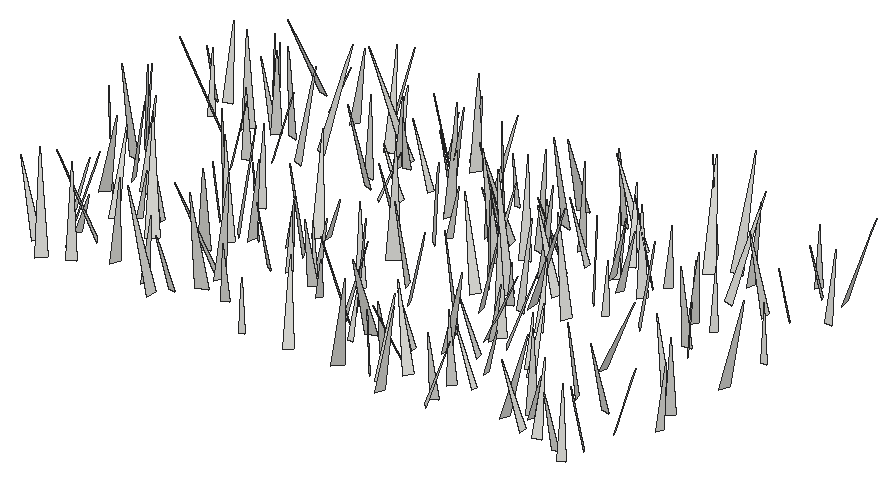
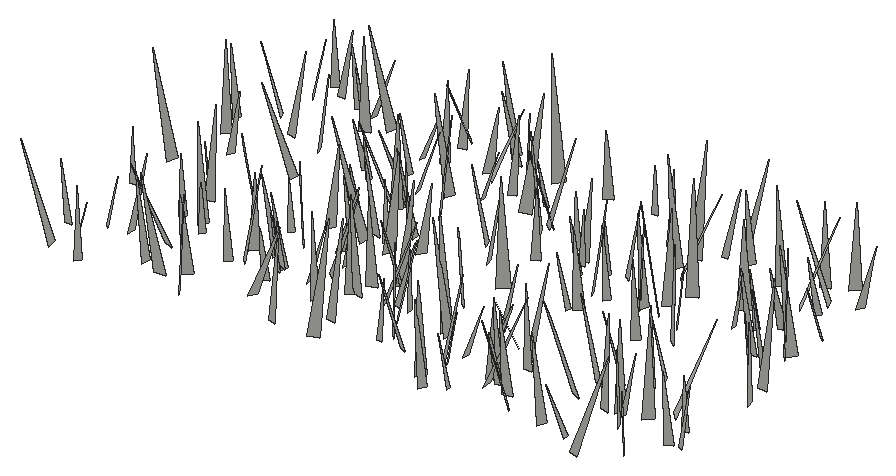
# SketchUp Ruby script. Lengths in inches.
U = 1.inch
M = Sketchup.active_model
def pt(a) = Geom::Point3d.new(a.map { |v| v * U })
def face(e, loops, mat)
  f = e.add_face(loops[0].map { |a| pt(a) })
  loops[1..].each { |l| e.add_face(l.map { |a| pt(a) }).erase! }
  f.material = f.back_material = mat if mat
  f
end
# faces: each face lists its corners as indices into pts; further lists are holes
def faces(e, pts, list, mat = nil) = list.each { |f| face(e, (f[0].is_a?(Array) ? f : [f]).map { |l| l.map { |i| pts[i] } }, mat) }
# xy, xz, yz: faces in a plane at the given z, y or x. An outline is a flat list of corners, or four numbers for a rectangle; further outlines are holes
def ring(l) = l.size == 4 ? [[l[0], l[1]], [l[2], l[1]], [l[2], l[3]], [l[0], l[3]]] : l.each_slice(2).to_a
def flat(e, list, mat, &to3) = list.each { |f| face(e, (f[0].is_a?(Array) ? f : [f]).map { |l| ring(l).map { |u, v| to3.(u, v) } }, mat) }
def xy(e, z, list, mat = nil) = flat(e, list, mat) { |x, y| [x, y, z] }
def xz(e, y, list, mat = nil) = flat(e, list, mat) { |x, z| [x, y, z] }
def yz(e, x, list, mat = nil) = flat(e, list, mat) { |y, z| [x, y, z] }
def lines(e, pts, list) = list.each { |a, b| e.add_line(pt(pts[a]), pt(pts[b])) }
# prism: a flat outline (further loops are holes) pulled along v
def prism(e, loops, v, mat = nil)
  f = face(e, loops, mat); d = Geom::Vector3d.new(v.map { |x| x * U })
  f.pushpull(f.normal.samedirection?(d) ? d.length : -d.length)
end
def box(e, o, s, mat = nil) = prism(e, [[o, [o[0] + s[0], o[1], o[2]], [o[0] + s[0], o[1] + s[1], o[2]], [o[0], o[1] + s[1], o[2]]]], [0, 0, s[2]], mat)
def at(x, y, z, deg = 0) = Geom::Transformation.translation(pt([x, y, z])) * Geom::Transformation.rotation(ORIGIN, Z_AXIS, deg.degrees)
def axes(o, x, y, z) = Geom::Transformation.new([*x, 0, *y, 0, *z, 0, *pt(o).to_a, 1])
def part(name) = M.definitions.add(name)
# library, detail: a bought-in or finely detailed component or shape, given as its bounding box
def library(name, o, s) = part(name).tap { |d| box(d.entities, o, s) }
def detail(e, o, s) = box(e.add_group.entities, o, s)
def put(e, d, t, mat = nil) = e.add_instance(d, t).tap { |i| i.material = mat if mat }
def group(e, t, mat = nil) = e.add_group.tap { |g| g.transformation = t; g.material = mat if mat }.entities
root = M.entities
c1 = part("fur_instance\#9")
p = [[0.8125,0,1.79],[0.67,-0.02,1.48],[0,-0.11,0],[0,0.11,0]]
faces(c1.entities,p,[[0,1,2,3]])
put(root,c1,axes([515.94,55.68,-21.66],[6.14943,-1.42717,1.61929],[-1.52874,-6.3314,0.22535],[-1.52376,0.59247,6.30885]))
put(root,c1,axes([507.93,57.48,-21.66],[6.18232,-5.30847,0.7026],[-5.32058,-6.21081,-0.10875],[-0.60412,0.37485,8.14795]))
put(root,c1,axes([544.28,55.85,-21.66],[-3.13208,3.88614,1.48189],[4.03166,3.29255,-0.11327],[1.02167,-1.07935,4.98991]))
put(root,c1,axes([542.07,57.4375,-21.66],[0.17037,-4.40384,1.04145],[-4.5148,-0.2364,-0.26107],[-0.30825,1.02847,4.3994]))
put(root,c1,axes([493.76,56.37,-21.66],[-0.42673,3.51272,1.26133],[3.73148,0.37463,0.21911],[-0.0791,-1.27778,3.53176]))
put(root,c1,axes([462.76,55.75,-21.66],[-5.4488,4.52209,1.619],[4.59694,5.6194,-0.22458],[1.39234,-0.85616,7.07731]))
put(root,c1,axes([479.05,57.01,-21.66],[-7.32255,-0.11088,1.35528],[-0.08815,7.44603,0.13288],[1.35695,-0.11461,7.32218]))
put(root,c1,axes([522.46,58.125,-21.66],[1.7038,-4.78318,1.39426],[-4.94528,-1.80274,-0.14134],[-0.60574,1.26373,5.0756]))
put(root,c1,axes([522.62,56.23,-21.66],[3.07177,3.42083,0.35758],[3.42072,-3.08846,0.16062],[-0.35863,-0.15826,4.59478]))
put(root,c1,axes([480.32,59.38,-21.66],[-0.08561,-4.51883,0.61864],[-4.55746,0.06047,-0.18896],[-0.17898,0.62161,4.51569]))
put(root,c1,axes([466.05,57.49,-21.66],[-2.20554,5.93145,2.00046],[6.2413,2.24627,0.22087],[0.47966,-1.95462,6.32437]))
put(root,c1,axes([500.67,56.875,-21.66],[-3.10471,5.12305,0.88051],[5.18598,3.12286,0.11631],[0.35573,-0.81381,5.98927]))
put(root,c1,axes([512.32,58.2,-21.66],[2.78644,2.89477,1.9564],[3.12581,-3.18339,0.25829],[-1.56092,-1.20736,4.00964]))
put(root,c1,axes([514.49,57.23,-21.66],[0.1573,5.82785,1.1486],[5.93788,-0.12389,-0.18455],[0.15705,-1.15268,5.82705]))
put(root,c1,axes([476.6,58.78,-21.66],[4.38951,-2.01268,1.547],[-2.15257,-4.58905,0.13732],[-1.34555,0.7756,4.82698]))
put(root,c1,axes([535.8,58.77,-21.66],[-4.77809,0.40303,0.49366],[0.4272,4.79644,0.21897],[0.47289,-0.2608,4.79006]))
put(root,c1,axes([544.7,59.71,-21.66],[-3.48684,-2.54111,1.02639],[-2.66037,3.53733,-0.28017],[0.65812,0.83597,4.30544]))
put(root,c1,axes([459.46,58.95,-21.66],[-4.99004,2.24313,0.58277],[2.2784,5.00139,0.2583],[0.42444,-0.4756,5.46492]))
put(root,c1,axes([538.38,58.38,-21.66],[-2.22109,4.73282,1.14399],[4.81333,2.32397,-0.26934],[0.73496,-0.91711,5.22114]))
put(root,c1,axes([531.96,60.09,-21.66],[6.74375,-1.56753,0.95704],[-1.61805,-6.79399,0.27364],[-0.86892,0.48558,6.91813]))
put(root,c1,axes([470.56,60.54,-21.66],[5.91489,-2.56905,1.81184],[-2.61095,-6.16477,-0.21752],[-1.75092,0.51416,6.44505]))
put(root,c1,axes([487.22,61.26,-21.66],[2.10827,-4.41232,0.88185],[-4.4927,-2.11805,0.1432],[-0.24874,0.85808,4.88803]))
put(root,c1,axes([482.97,61.99,-21.66],[2.46891,-7.20313,1.70316],[-7.36136,-2.57683,-0.22704],[-0.77207,1.53499,7.61111]))
put(root,c1,axes([514.81,62.16,-21.66],[-3.4454,-3.89131,0.03074],[-3.88746,3.44363,0.20759],[0.17579,-0.11462,5.19326]))
put(root,c1,axes([534.76,61.78,-21.66],[3.71508,-1.29272,0.27873],[-1.28155,-3.72443,-0.19222],[-0.32626,-0.0905,3.92887]))
put(root,c1,axes([462.98,60.62,-21.66],[6.72571,2.73267,0.89443],[2.78268,-6.75899,-0.27437],[-0.72399,-0.59256,7.25447]))
put(root,c1,axes([521.89,62.25,-21.66],[4.08918,-3.36848,1.98263],[-3.52303,-4.41912,-0.24183],[-1.69286,1.05996,5.29241]))
put(root,c1,axes([510.38,63.55,-21.66],[2.722,-4.21365,0.18087],[-4.20663,-2.72794,-0.24377],[-0.30292,0.01939,5.01046]))
put(root,c1,axes([465.27,63.52,-21.66],[-5.5722,-4.07145,0.43281],[-4.071,5.58734,0.1482],[0.43699,0.13539,6.89957]))
put(root,c1,axes([516.1,61,-21.66],[-4.785,3.6619,0.62252],[3.69492,4.79647,0.18627],[0.38032,-0.52686,6.02254]))
put(root,c1,axes([534.39,62.39,-21.66],[-1.98157,5.41612,3.08152],[6.10168,2.34277,-0.19399],[1.26474,-2.81671,5.76397]))
put(root,c1,axes([462.39,63.51,-21.66],[3.14021,-1.95272,0.11029],[-1.95573,-3.13292,0.21476],[0.01996,0.24059,3.6916]))
put(root,c1,axes([506.39,66.02,-21.66],[2.6634,-7.09113,0.13913],[-7.08626,-2.66678,-0.26525],[-0.29724,0.03689,7.57017]))
put(root,c1,axes([524.63,63.32,-21.66],[-3.98782,0.86871,0.11292],[0.87287,3.98492,0.16912],[0.07423,-0.18933,4.07783]))
put(root,c1,axes([505.36,63.11,-21.66],[0.0321,3.78164,0.61426],[3.82721,-0.05969,0.16749],[-0.17489,-0.6122,3.77806]))
put(root,c1,axes([483.15,65.27,-21.66],[6.93717,-2.75986,2.51351],[-2.97128,-7.29338,0.19237],[-2.25967,1.11744,7.46352]))
put(root,c1,axes([481.44,66.5,-21.66],[-5.39414,-3.77764,0.22745],[-3.78403,5.38986,-0.22257],[0.05845,0.31282,6.58162]))
put(root,c1,axes([501.96,66.91,-21.66],[-3.86878,-4.9807,0.99535],[-5.05831,3.89149,-0.18804],[0.45997,0.9025,6.30392]))
put(root,c1,axes([544.89,65.53,-21.66],[4.65489,2.00226,0.76997],[2.06003,-4.68544,-0.26978],[-0.59848,-0.55448,5.06006]))
put(root,c1,axes([512.64,66.44,-21.66],[-3.89073,-0.42692,0.42553],[-0.44504,3.90915,-0.14719],[0.40654,0.19356,3.91132]))
put(root,c1,axes([523.32,67.25,-21.66],[3.83276,-0.80553,0.30542],[-0.78769,-3.84079,-0.24507],[-0.34886,-0.17786,3.90882]))
put(root,c1,axes([540.79,68.76,-21.66],[-1.08369,-5.40972,1.03151],[-5.49173,1.14023,0.21038],[0.41232,0.96864,5.51318]))
put(root,c1,axes([501.6,66.56,-21.66],[3.62165,4.35293,0.90177],[4.41878,-3.65214,-0.11732],[-0.48531,-0.76904,5.66132]))
put(root,c1,axes([477.28,69.61,-21.66],[4.02071,-6.30995,0.86141],[-6.36147,-4.02715,0.19326],[-0.29869,0.83076,7.47959]))
put(root,c1,axes([516.22,68.47,-21.66],[6.40795,-1.734,1.03011],[-1.73088,-6.48917,-0.15614],[-1.03535,0.11648,6.63658]))
put(root,c1,axes([495.57,69.25,-21.66],[2.79472,-2.37927,0.19168],[-2.37504,-2.80125,-0.14262],[-0.23842,0.01542,3.66757]))
put(root,c1,axes([458.3,67.97,-21.66],[2.21445,2.95218,0.72503],[3.03203,-2.20951,-0.26401],[-0.21871,-0.73996,3.68096]))
put(root,c1,axes([501.79,68.63,-21.66],[5.69134,3.55142,2.30083],[3.82093,-5.97012,-0.23634],[-1.81848,-1.42926,6.70433]))
put(root,c1,axes([535.89,69.44,-21.66],[4.40996,1.53054,2.75088],[1.88618,-5.07543,-0.19988],[-2.52036,-1.1203,4.66373]))
put(root,c1,axes([548.86,69.37,-21.66],[4.44334,-1.86269,1.64457],[-2.02269,-4.66849,0.17731],[-1.44323,0.80817,4.81471]))
put(root,c1,axes([520.02,69.99,-21.66],[-4.58656,-0.99691,0.53395],[-0.9871,4.61746,0.14195],[0.55187,-0.02624,4.69151]))
put(root,c1,axes([493.13,71.04,-21.66],[2.16413,-4.87719,1.14426],[-4.95965,-2.26151,-0.2591],[-0.70577,0.93721,5.32947]))
put(root,c1,axes([470.29,68.15,-21.66],[-5.1988,6.07272,1.14347],[6.1224,5.26442,-0.12263],[0.83765,-0.78798,7.99315]))
put(root,c1,axes([486.35,70.99,-21.66],[-2.7828,-3.97435,1.2381],[-4.07565,2.90431,0.16237],[0.84701,0.91751,4.84903]))
put(root,c1,axes([465.95,71.1,-21.66],[3.13443,-2.25979,0.73802],[-2.32723,-3.16608,0.18952],[-0.4851,0.5876,3.85946]))
put(root,c1,axes([463.53,68.97,-21.66],[-2.14385,5.53708,0.23418],[5.53457,2.15208,-0.21752],[0.2875,-0.13964,5.93364]))
put(root,c1,axes([528.35,69.8,-21.66],[-1.52341,4.48001,0.30788],[4.47725,1.54034,-0.26007],[0.34571,-0.20714,4.72479]))
put(root,c1,axes([492.76,71.94,-21.66],[-0.42877,3.87256,1.55947],[4.17346,0.35848,0.25729],[-0.1042,-1.57711,3.88772]))
put(root,c1,axes([526.67,71.23,-21.66],[-1.83169,3.1238,0.57494],[3.14275,1.87858,-0.19441],[0.4602,-0.39568,3.61599]))
put(root,c1,axes([468.62,72.25,-21.66],[-3.8802,0.07929,1.10053],[0.11582,4.03064,0.11798],[1.09728,-0.14508,3.87922]))
put(root,c1,axes([488.75,71.93,-21.66],[-3.06481,2.41196,1.362],[2.48233,3.29293,-0.24563],[1.22908,-0.63618,3.89234]))
put(root,c1,axes([458.44,73.67,-21.66],[5.57249,-4.36069,0.56036],[-4.38496,-5.5781,0.19774],[-0.31889,0.50141,7.07313]))
put(root,c1,axes([547.42,73.18,-21.66],[-3.8078,3.44308,3.43375],[4.19662,4.52997,0.11149],[2.45637,-2.40193,5.13242]))
put(root,c1,axes([513.98,73.22,-21.66],[-6.04607,-3.24149,2.31572],[-3.3744,6.40425,0.15438],[2.11738,0.95032,6.85845]))
put(root,c1,axes([478.23,73.08,-21.66],[-4.52139,5.22079,2.42729],[5.56937,4.74843,0.161],[1.45961,-1.94607,6.90462]))
put(root,c1,axes([459.07,74.31,-21.66],[-4.9247,-5.05159,2.9073],[-5.39927,5.38751,0.21521],[2.19519,1.91829,7.05159]))
put(root,c1,axes([518.82,74.01,-21.66],[4.01363,-0.60213,1.19124],[-0.70216,-4.16285,0.26162],[-1.13516,0.446,4.0501]))
put(root,c1,axes([491.41,74.21,-21.66],[3.83893,-0.81047,1.08867],[-0.8917,-3.9684,0.19003],[-1.0232,0.41758,3.91895]))
put(root,c1,axes([518.03,73.83,-21.66],[5.44846,0.74036,0.07595],[0.73692,-5.44519,0.21553],[-0.10422,0.20337,5.4943]))
put(root,c1,axes([521.3,73.87,-21.66],[4.74716,3.3592,0.52437],[3.38285,-4.75689,-0.1518],[-0.33985,-0.42721,5.81349]))
put(root,c1,axes([480.22,75.41,-21.66],[5.9168,-1.45412,1.7202],[-1.44139,-6.15974,-0.24915],[-1.73089,0.15879,6.08776]))
put(root,c1,axes([498.02,74.4,-21.66],[2.13883,-4.28297,3.06723],[-5.00629,-2.68295,-0.2554],[-1.63976,2.60467,4.7805]))
put(root,c1,axes([505.16,74.95,-21.66],[5.01565,1.80166,1.23073],[1.89818,-5.12441,-0.23415],[-1.07592,-0.64182,5.32428]))
put(root,c1,axes([480.64,75.9,-21.66],[-3.25997,-4.21096,1.97124],[-4.4396,3.53441,0.20814],[1.38129,1.42168,5.3213]))
put(root,c1,axes([484.92,76.76,-21.66],[3.8804,-2.67072,0.47699],[-2.66948,-3.90717,-0.15997],[-0.48385,0.13783,4.70793]))
put(root,c1,axes([487.4,76.46,-21.66],[-5.57513,-2.9786,1.92177],[-3.03694,5.86084,0.2736],[1.82819,0.65252,6.315]))
put(root,c1,axes([519.27,75.08,-21.66],[-5.69,4.35692,2.08043],[4.49689,5.95288,-0.16772],[1.75752,-1.1258,7.16454]))
put(root,c1,axes([477.97,75.39,-21.66],[5.88152,4.86813,2.28116],[5.13014,-6.09312,-0.22398],[-1.60749,-1.63397,7.63157]))
put(root,c1,axes([473.96,76.7,-21.66],[-3.08736,-2.6391,1.38175],[-2.74426,3.29386,0.15946],[1.15895,0.7691,4.05847]))
put(root,c1,axes([534.06,76.74,-21.66],[6.32443,-0.86949,0.03215],[-0.87008,-6.31952,0.24926],[0.00213,0.25131,6.37905]))
put(root,c1,axes([462.55,76.25,-21.66],[-0.45657,6.34549,1.8425],[6.59681,0.54314,-0.23589],[0.37708,-1.81886,6.35752]))
put(root,c1,axes([543.77,76.92,-21.66],[-4.87029,1.64927,0.93909],[1.65484,4.95663,-0.12272],[0.92923,-0.18296,5.1405]))
put(root,c1,axes([502.15,78.37,-21.66],[-5.31437,-1.63311,1.48269],[-1.72892,5.48589,-0.1545],[1.36976,0.58821,5.55749]))
put(root,c1,axes([459.34,78.15,-21.66],[5.12051,1.66894,1.66295],[1.70709,-5.37015,0.13306],[-1.62376,-0.38277,5.38398]))
put(root,c1,axes([513.03,79.12,-21.66],[5.83146,1.27805,1.15338],[1.33487,-5.92923,-0.17895],[-1.08712,-0.42484,5.96719]))
put(root,c1,axes([472.03,80.09,-21.66],[3.78368,4.97369,3.03573],[5.56614,-4.15585,-0.12867],[-1.72376,-2.50217,6.24798]))
put(root,c1,axes([522,79.2,-21.66],[-1.31854,4.49628,0.43937],[4.51767,1.31381,0.11263],[0.01505,-0.45333,4.68427]))
put(root,c1,axes([456.17,82.26,-21.66],[-0.95753,-7.17721,1.84222],[-7.39469,1.0444,0.22542],[0.47406,1.79439,7.23729]))
put(root,c1,axes([487.26,81.5,-21.66],[3.61055,-0.61097,0.20103],[-0.59508,-3.6081,-0.27795],[-0.24409,-0.24103,3.65131]))
put(root,c1,axes([515.02,82.45,-21.66],[2.03296,-3.43324,0.36978],[-3.45285,-2.01606,0.26469],[0.04074,0.45292,3.9812]))
put(root,c1,axes([548.43,82.57,-21.66],[6.87118,-2.4682,1.14103],[-2.53265,-6.93781,0.24398],[-0.98977,0.61792,7.29696]))
put(root,c1,axes([486.15,80.77,-21.66],[-3.98192,5.65644,1.02142],[5.69703,4.04883,-0.21229],[0.76316,-0.7113,6.91418]))
put(root,c1,axes([476.07,82.22,-21.66],[-2.39493,4.93051,2.15105],[5.27679,2.61079,-0.10925],[1.04521,-1.88321,5.4803]))
put(root,c1,axes([496.72,82.32,-21.66],[4.92232,-5.34816,3.43981],[-5.97476,-5.37881,0.1869],[-2.17654,2.67018,7.26616]))
put(root,c1,axes([517.0625,81.81,-21.66],[1.06492,5.99669,1.55027],[6.17359,-1.15473,0.22589],[-0.50038,-1.48458,6.08632]))
put(root,c1,axes([509.93,81.82,-21.66],[-5.57386,3.34507,0.61319],[3.34749,5.6042,-0.14346],[0.5998,-0.19191,6.49898]))
put(root,c1,axes([517.41,83.75,-21.66],[8.28106,0.30024,0.90595],[0.31898,-8.32832,-0.15571],[-0.89952,-0.18935,8.28504]))
put(root,c1,axes([510.06,84.21,-21.66],[4.77754,4.17311,2.72058],[4.61145,-5.13068,-0.22808],[-1.8844,-1.97551,6.33938]))
put(root,c1,axes([522.66,83.89,-21.66],[-6.31107,2.62453,1.38258],[2.63294,6.45317,-0.23139],[1.36651,-0.31261,6.83112]))
put(root,c1,axes([513.21,84.08,-21.66],[-7.4138,3.10521,1.79195],[3.13289,7.61249,-0.22981],[1.74312,-0.47482,8.03455]))
put(root,c1,axes([456.03,84.6875,-21.66],[3.99026,4.07334,2.14881],[4.32029,-4.29562,0.12027],[-1.59518,-1.44473,5.70086]))
put(root,c1,axes([455.0625,86.07,-21.66],[-4.85936,-1.80324,2.4582],[-1.94231,5.39639,0.11902],[2.34986,0.73149,5.18178]))
put(root,c1,axes([539.9375,86.04,-21.66],[-2.43911,-2.15453,1.73505],[-2.51562,2.68975,-0.19638],[1.15067,1.31336,3.24849]))
put(root,c1,axes([538.45,87.67,-21.66],[0.4786,-6.17329,1.68247],[-6.39725,-0.42884,0.2463],[0.12453,1.69584,6.18692]))
put(root,c1,axes([525.85,87.54,-21.66],[-2.23187,2.81976,1.51549],[3.01775,2.4697,-0.15093],[1.06816,-1.08561,3.59298]))
put(root,c1,axes([466.8,87.88,-21.66],[4.26525,2.34746,1.0733],[2.44325,-4.34035,-0.2164],[-0.83252,-0.71113,4.86375]))
put(root,c1,axes([518.05,87.66,-21.66],[-5.4054,2.23783,0.44972],[2.26041,5.40869,0.2551],[0.31726,-0.40826,5.84475]))
put(root,c1,axes([530.82,87.88,-21.66],[-3.67972,-3.6806,3.42599],[-4.33109,4.47676,0.15761],[2.55458,2.28831,5.20214]))
put(root,c1,axes([498.01,88.61,-21.66],[3.30572,4.13092,2.03155],[4.38871,-3.58299,0.14433],[-1.38957,-1.489,5.28881]))
put(root,c1,axes([490.24,90.58,-21.66],[-1.40933,-4.17013,0.64925],[-4.20295,1.44894,0.18319],[0.38311,0.55526,4.39803]))
put(root,c1,axes([522.62,89.11,-21.66],[3.82157,4.19761,2.25189],[4.45533,-4.17126,0.21447],[-1.68552,-1.50865,5.67259]))
put(root,c1,axes([507.04,89.48,-21.66],[-7.37907,1.498,2.27835],[1.63074,7.6926,0.22378],[2.18531,-0.6822,7.52626]))
put(root,c1,axes([467.23,90.51,-21.66],[1.77747,-4.94769,1.74658],[-5.22789,-1.82695,0.145],[-0.44649,1.69476,5.25529]))
put(root,c1,axes([515.35,90.03,-21.66],[-3.60239,-0.15597,0.87969],[-0.19043,3.7046,-0.12301],[0.87288,0.16452,3.60367]))
put(root,c1,axes([548.5,90.3,-21.66],[-0.06677,3.94377,1.582],[4.24655,0.00562,0.16522],[-0.15123,-1.5834,3.94087]))
put(root,c1,axes([498.66,90.79,-21.66],[3.79566,-1.87078,0.73995],[-1.92959,-3.83243,0.2087],[-0.56925,0.51676,4.2265]))
put(root,c1,axes([513.58,90.52,-21.66],[6.28963,-0.96384,2.1084],[-1.07131,-6.61487,0.17192],[-2.05588,0.49827,6.36073]))
put(root,c1,axes([506.45,90.0625,-21.66],[2.03381,4.83721,0.83738],[4.90479,-2.04045,-0.1258],[-0.20703,-0.82108,5.24587]))
put(root,c1,axes([535.49,92.67,-21.66],[5.23742,-3.794,0.7561],[-3.79638,-5.28528,-0.22367],[-0.74406,0.26094,6.46336]))
put(root,c1,axes([515.09,93.07,-21.66],[-2.82637,-5.01502,0.69558],[-5.06125,2.81969,-0.23605],[0.13409,0.7222,5.75179]))
put(root,c1,axes([460.44,94.08,-21.66],[-5.16383,-5.19186,0.43743],[-5.2089,5.15828,-0.26709],[0.11856,0.49863,7.31773]))
put(root,c1,axes([469.76,92.46,-21.66],[4.69401,2.26049,0.88712],[2.32694,-4.7392,-0.23643],[-0.69438,-0.60059,5.20458]))
put(root,c1,axes([504,93.98,-21.66],[-1.28236,-4.10189,0.60594],[-4.14572,1.27987,-0.10961],[0.07509,0.61118,4.29626]))
put(root,c1,axes([523.41,93.34,-21.66],[4.86131,-2.02952,0.59697],[-2.06386,-4.87843,0.22145],[-0.46454,0.43544,5.26329]))
put(root,c1,axes([538.64,92.7,-21.66],[-2.37433,3.47563,1.70417],[3.72029,2.6012,-0.12184],[1.06942,-1.33243,4.20745]))
put(root,c1,axes([483.01,94.51,-21.66],[-2.27159,-6.08211,1.19958],[-6.16809,2.34544,0.21162],[0.62109,1.04786,6.48903]))
put(root,c1,axes([509.51,92.15,-21.66],[-2.53684,6.34204,1.9532],[6.60869,2.60398,0.12835],[0.60133,-1.86275,6.82939]))
put(root,c1,axes([486.03,92.73,-21.66],[2.19151,2.85606,0.09461],[2.85445,-2.18225,-0.24214],[0.13471,-0.22234,3.59182]))
put(root,c1,axes([510.63,95.16,-21.66],[2.81621,-4.35059,0.38195],[-4.36621,-2.81499,0.12899],[-0.09891,0.39082,5.18093]))
put(root,c1,axes([502.12,93.91,-21.66],[3.8396,0.83392,1.68617],[0.96833,-4.16197,-0.14664],[-1.61273,-0.51356,3.92638]))
put(root,c1,axes([505.58,94.53,-21.66],[-6.60705,-1.5953,0.55499],[-1.61141,6.62494,-0.14037],[0.50631,0.26714,6.79547]))
put(root,c1,axes([488.34,94.29,-21.66],[-3.79909,0.62191,0.11225],[0.62576,3.79759,0.13861],[0.08831,-0.15497,3.84716]))
put(root,c1,axes([526.51,93.88,-21.66],[-4.60516,3.74944,1.60687],[3.84875,4.79672,-0.16237],[1.35183,-0.88372,5.93628]))
put(root,c1,axes([472.625,93.79,-21.66],[2.70818,5.99392,1.73773],[6.22026,-2.74585,-0.22279],[-0.5051,-1.67756,6.57356]))
put(root,c1,axes([534.09,94.58,-21.66],[2.31719,-2.3997,1.71249],[-2.74416,-2.55172,0.13746],[-1.07739,1.33819,3.33302]))
put(root,c1,axes([520.69,95.32,-21.66],[4.88822,-0.89007,0.63341],[-0.87396,-4.92864,-0.18113],[-0.65546,-0.06625,4.96529]))
put(root,c1,axes([495.4,95.01,-21.66],[7.52534,-2.11015,2.94691],[-2.32099,-8.02168,0.183],[-2.78389,0.98374,7.81345]))
put(root,c1,axes([509.59,94.875,-21.66],[-1.17344,-6.36654,3.3674],[-7.15717,1.41187,0.17527],[0.80444,3.27459,6.4714]))
put(root,c1,axes([516.35,95.89,-21.66],[-4.66446,-0.17714,0.77084],[-0.14932,4.72517,0.1823],[0.77671,-0.15541,4.66426]))
put(root,c1,axes([494.57,95.84,-21.66],[7.78387,0.2727,2.09642],[0.3333,-8.05673,-0.18953],[-2.08764,-0.26953,7.78634]))
put(root,c1,axes([525.74,96.8,-21.66],[4.20893,3.73459,3.7879],[4.59902,-4.98198,-0.19834],[-2.67289,-2.69131,5.62342]))
put(root,c1,axes([501.75,96.77,-21.66],[-4.7875,-3.33897,1.34753],[-3.4677,4.87923,-0.23006],[0.96934,0.96392,5.83232]))
put(root,c1,axes([481.63,96.44,-21.66],[0.33576,5.45677,2.6197],[6.05197,-0.25349,-0.24764],[0.11336,-2.62894,5.46148]))
put(root,c1,axes([520.93,96.17,-21.66],[1.65832,3.59632,1.35209],[3.82471,-1.68517,-0.20869],[-0.36513,-1.31848,3.95475]))
put(root,c1,axes([462.46,96.79,-21.66],[-4.98307,4.13485,3.06586],[4.6284,5.46651,0.15019],[2.25263,-2.08511,6.47344]))
put(root,c1,axes([521.05,95.57,-21.66],[-1.86481,4.13252,0.34952],[4.14724,1.85655,0.17621],[-0.01744,-0.39104,4.53037]))
put(root,c1,axes([456.92,96.39,-21.66],[-1.17354,4.22506,1.16991],[4.38332,1.15287,0.2334],[0.0799,-1.19029,4.3788]))
put(root,c1,axes([466.07,97.78,-21.66],[4.61817,-3.87726,2.02523],[-4.05143,-4.90172,-0.14567],[-1.64942,1.18414,6.02822]))
put(root,c1,axes([527.37,97.9,-21.66],[-2.45808,3.26284,2.53045],[3.74921,2.99751,-0.22312],[1.72995,-1.86016,4.07903]))
put(root,c1,axes([468.05,98.375,-21.66],[-1.72933,-6.01967,2.37326],[-6.41752,1.90965,0.16749],[0.82719,2.23073,6.26091]))
put(root,c1,axes([465.38,98.1,-21.66],[-4.97388,0.03891,0.99351],[0.0174,5.07103,-0.11152],[0.99411,0.10595,4.97278]))
put(root,c1,axes([513.2,98.7,-21.66],[5.69837,-0.41307,2.53776],[-0.52377,-6.22748,0.16244],[-2.51724,0.36068,5.71101]))
put(root,c1,axes([489.6875,98.41,-21.66],[-4.67921,0.76999,0.1435],[0.76372,4.67821,-0.1991],[0.17382,0.17327,4.73796]))
put(root,c1,axes([454.9,99.89,-21.66],[-2.14945,-3.42966,1.0737],[-3.50191,2.27993,0.27214],[0.80747,0.75821,4.03839]))
put(root,c1,axes([541.13,99.65,-21.66],[-5.71627,0.02456,1.51927],[0.09668,5.9079,0.26822],[1.51639,-0.28405,5.71003]))
put(root,c1,axes([483.88,101.02,-21.66],[1.95757,-4.55386,0.31612],[-4.56359,-1.94437,0.25034],[0.10577,0.38911,4.95045]))
put(root,c1,axes([473.11,97.69,-21.66],[2.96798,6.81466,1.03357],[6.887,-2.97737,-0.1458],[-0.27767,-1.00619,7.4315]))
put(root,c1,axes([499.75,100.04,-21.66],[4.37424,4.04681,2.79179],[4.54542,-4.75288,-0.23239],[-1.87347,-2.08284,5.95454]))
put(root,c1,axes([482.98,100.27,-21.66],[5.23095,-0.44242,1.6949],[-0.413,-5.49862,-0.16069],[-1.70231,-0.02548,5.24716]))
put(root,c1,axes([544.28,100.5,-21.66],[-2.57629,-2.49445,0.93197],[-2.62206,2.60252,-0.28257],[0.46438,0.85602,3.57488]))
put(root,c1,axes([464.22,100.34,-21.66],[4.38059,2.58911,2.20412],[2.75267,-4.81057,0.18002],[-1.99611,-0.9519,5.08534]))
put(root,c1,axes([508.18,101.77,-21.66],[-1.31696,-6.51866,1.83434],[-6.75362,1.40125,0.13086],[0.49623,1.77078,6.64907]))
put(root,c1,axes([520.74,98.98,-21.66],[-2.1836,4.82414,0.14178],[4.82373,2.17653,0.23433],[-0.15514,-0.2257,5.29014]))
put(root,c1,axes([490.73,101.48,-21.66],[3.77255,3.78798,3.73229],[4.48771,-4.72284,0.25719],[-2.85294,-2.4201,5.33992]))
put(root,c1,axes([456.43,100.26,-21.66],[-1.35199,5.16754,1.66066],[5.39955,1.4549,-0.13134],[0.55327,-1.57128,5.33986]))
put(root,c1,axes([490.39,101.25,-21.66],[-3.18222,-1.83698,0.96818],[-1.93012,3.2701,-0.13938],[0.76583,0.60852,3.67173]))
put(root,c1,axes([500.37,102.0625,-21.66],[0.0054,-4.02258,1.09842],[-4.16704,0.03516,0.14925],[0.15324,1.09787,4.01982]))
put(root,c1,axes([483.22,102.39,-21.66],[-7.85705,-0.88135,0.16267],[-0.88597,7.85465,-0.23661],[0.1352,0.25331,7.90278]))
put(root,c1,axes([535.55,99.43,-21.66],[2.14003,7.20036,0.0672],[7.19519,-2.14104,0.27303],[-0.28086,0.01341,7.50668]))
put(root,c1,axes([482.07,101.46,-21.66],[-0.89857,4.82904,0.37817],[4.8418,0.88433,0.21213],[-0.14006,-0.41036,4.90735]))
put(root,c1,axes([496.72,102.02,-21.66],[2.68485,5.08236,0.90598],[5.15716,-2.6868,-0.21076],[-0.23424,-0.9002,5.74408]))
put(root,c1,axes([519.68,102.72,-21.66],[-6.207,1.9177,0.03314],[1.91765,6.20287,0.22937],[-0.03607,-0.22893,6.49244]))
put(root,c1,axes([507.38,106.23,-21.66],[2.10072,-7.09935,0.00934],[-7.09522,-2.09917,0.25546],[0.24231,0.08144,7.39923]))
put(root,c1,axes([548.48,102.87,-21.66],[0.70725,4.81258,1.31899],[4.97344,-0.78845,0.21001],[-0.40688,-1.27212,4.85974]))
put(root,c1,axes([479.67,102.85,-21.66],[-1.61925,6.67608,1.38838],[6.8184,1.60284,0.24489],[0.08425,-1.4073,6.86528]))
put(root,c1,axes([535.05,104.44,-21.66],[5.91491,-0.67607,1.90084],[-0.77835,-6.19702,0.21795],[-1.8613,0.44302,5.94943]))
put(root,c1,axes([459.38,105.34,-21.66],[3.09242,2.58599,1.68004],[2.84079,-3.31463,-0.12697],[-1.19992,-1.18273,4.02918]))
put(root,c1,axes([471.875,105.9,-21.66],[4.94298,-3.20176,1.42299],[-3.34359,-5.04595,0.26096],[-1.0472,0.99819,5.88356]))
put(root,c1,axes([529.19,103.69,-21.66],[-4.20767,6.2047,0.57896],[6.20765,4.23458,-0.26697],[0.54635,-0.32858,7.49209]))
put(root,c1,axes([491,105.6875,-21.66],[-5.47966,3.19166,2.7493],[3.39794,6.01513,-0.2105],[2.48986,-1.18473,6.33791]))
put(root,c1,axes([513.71,106.46,-21.66],[-1.84582,-5.09705,1.94608],[-5.40108,1.99766,0.10933],[0.77171,1.78987,5.41987]))
put(root,c1,axes([486.34,106.12,-21.66],[3.55375,0.65284,0.74182],[0.70307,-3.6162,-0.18565],[-0.69441,-0.32026,3.60844]))
put(root,c1,axes([477.64,105.2,-21.66],[4.5925,4.65986,1.11021],[4.70947,-4.6734,0.13435],[-0.87619,-0.69491,6.5412]))
put(root,c1,axes([464.23,109.24,-21.66],[-1.51656,-6.50321,0.08888],[-6.50028,1.51258,-0.24097],[-0.21452,0.14123,6.67335]))
put(root,c1,axes([467.46,106.64,-21.66],[3.69637,0.13401,0.11411],[0.12786,-3.69317,0.19555],[-0.12096,0.19138,3.69362]))
put(root,c1,axes([489.01,107.88,-21.66],[4.9839,-2.53795,0.76874],[-2.53211,-5.04073,-0.2255],[-0.78777,0.14572,5.58834]))
put(root,c1,axes([543.72,107.57,-21.66],[-3.07283,-1.79032,0.75021],[-1.87261,3.10397,-0.26279],[0.51124,0.60869,3.54662]))
put(root,c1,axes([531.77,105.75,-21.66],[-0.24232,8.0833,1.63068],[8.24361,0.27788,-0.15248],[0.20433,-1.625,8.08549]))
put(root,c1,axes([527.19,107.71,-21.66],[-5.46878,-3.64969,2.6695],[-4.02035,5.84198,-0.2491],[2.0696,1.70441,6.57007]))
put(root,c1,axes([546.8,108.14,-21.66],[7.02887,1.41814,0.69885],[1.44367,-7.05544,-0.2028],[-0.64447,-0.3379,7.16763]))
put(root,c1,axes([541.86,109.3,-21.66],[3.93082,-2.70083,1.38603],[-2.7651,-4.12134,-0.18897],[-1.2529,0.6221,4.76552]))
